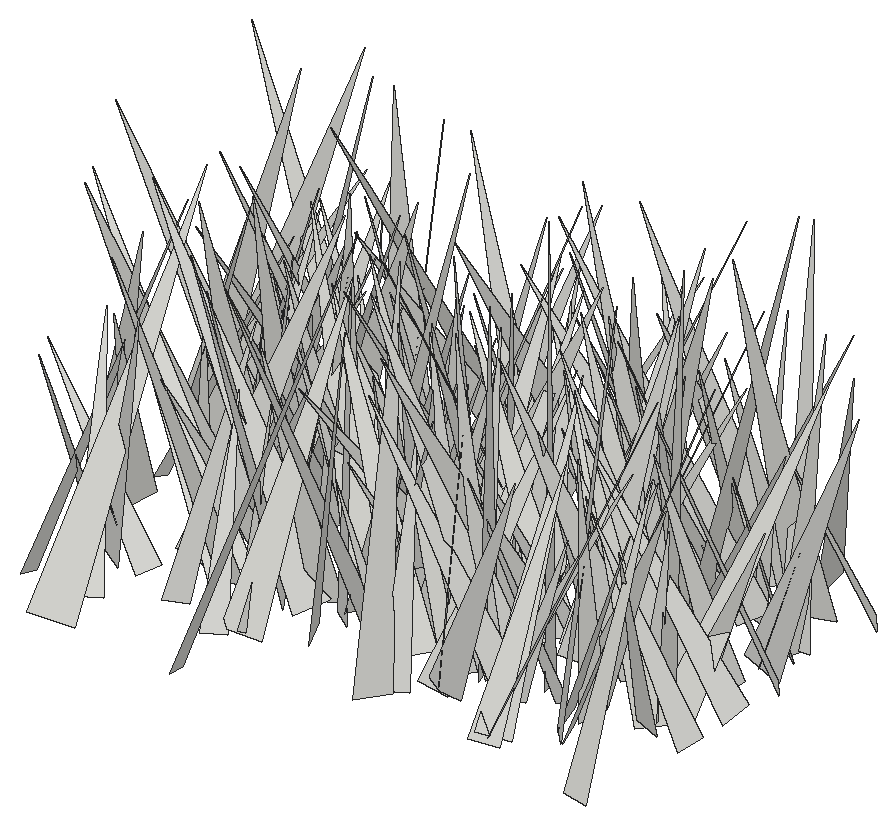
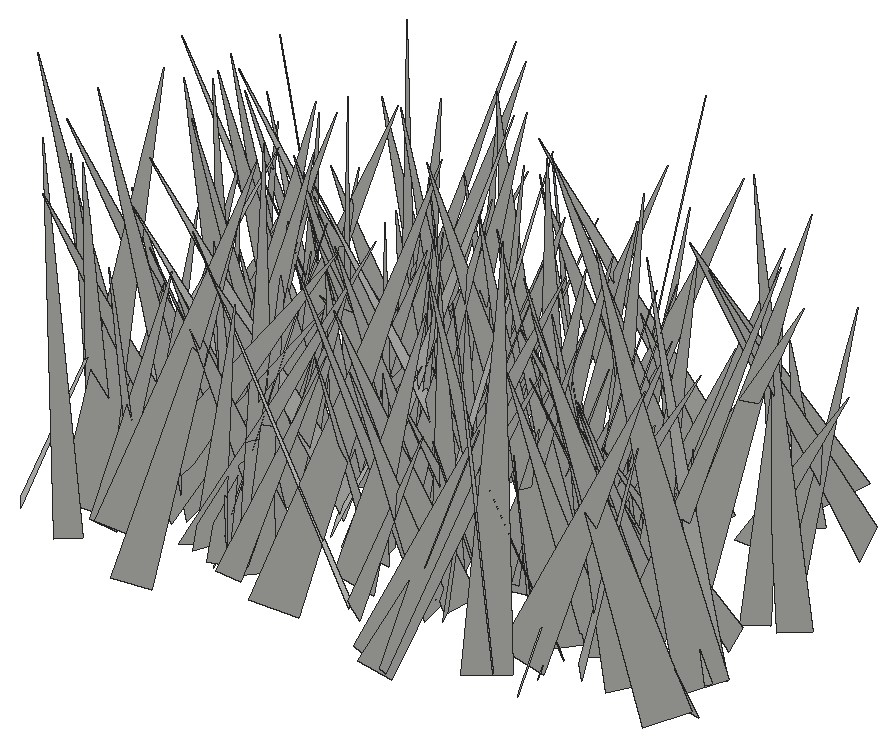
# SketchUp Ruby script. Lengths in inches.
U = 1.inch
M = Sketchup.active_model
def pt(a) = Geom::Point3d.new(a.map { |v| v * U })
def face(e, loops, mat)
  f = e.add_face(loops[0].map { |a| pt(a) })
  loops[1..].each { |l| e.add_face(l.map { |a| pt(a) }).erase! }
  f.material = f.back_material = mat if mat
  f
end
# faces: each face lists its corners as indices into pts; further lists are holes
def faces(e, pts, list, mat = nil) = list.each { |f| face(e, (f[0].is_a?(Array) ? f : [f]).map { |l| l.map { |i| pts[i] } }, mat) }
# xy, xz, yz: faces in a plane at the given z, y or x. An outline is a flat list of corners, or four numbers for a rectangle; further outlines are holes
def ring(l) = l.size == 4 ? [[l[0], l[1]], [l[2], l[1]], [l[2], l[3]], [l[0], l[3]]] : l.each_slice(2).to_a
def flat(e, list, mat, &to3) = list.each { |f| face(e, (f[0].is_a?(Array) ? f : [f]).map { |l| ring(l).map { |u, v| to3.(u, v) } }, mat) }
def xy(e, z, list, mat = nil) = flat(e, list, mat) { |x, y| [x, y, z] }
def xz(e, y, list, mat = nil) = flat(e, list, mat) { |x, z| [x, y, z] }
def yz(e, x, list, mat = nil) = flat(e, list, mat) { |y, z| [x, y, z] }
def lines(e, pts, list) = list.each { |a, b| e.add_line(pt(pts[a]), pt(pts[b])) }
# prism: a flat outline (further loops are holes) pulled along v
def prism(e, loops, v, mat = nil)
  f = face(e, loops, mat); d = Geom::Vector3d.new(v.map { |x| x * U })
  f.pushpull(f.normal.samedirection?(d) ? d.length : -d.length)
end
def box(e, o, s, mat = nil) = prism(e, [[o, [o[0] + s[0], o[1], o[2]], [o[0] + s[0], o[1] + s[1], o[2]], [o[0], o[1] + s[1], o[2]]]], [0, 0, s[2]], mat)
def at(x, y, z, deg = 0) = Geom::Transformation.translation(pt([x, y, z])) * Geom::Transformation.rotation(ORIGIN, Z_AXIS, deg.degrees)
def axes(o, x, y, z) = Geom::Transformation.new([*x, 0, *y, 0, *z, 0, *pt(o).to_a, 1])
def part(name) = M.definitions.add(name)
# library, detail: a bought-in or finely detailed component or shape, given as its bounding box
def library(name, o, s) = part(name).tap { |d| box(d.entities, o, s) }
def detail(e, o, s) = box(e.add_group.entities, o, s)
def put(e, d, t, mat = nil) = e.add_instance(d, t).tap { |i| i.material = mat if mat }
def group(e, t, mat = nil) = e.add_group.tap { |g| g.transformation = t; g.material = mat if mat }.entities
root = M.entities
c1 = part("fur_instance\#9")
p = [[0.8125,0,1.79],[0.67,-0.02,1.48],[0,-0.11,0],[0,0.11,0]]
faces(c1.entities,p,[[0,1,2,3]])
put(root,c1,axes([550.24,70.07,-21.86],[1.54833,5.59255,0.52827],[5.59137,-1.58705,0.41342],[-0.54067,-0.39706,5.78818]))
put(root,c1,axes([542.11,73.05,-21.86],[2.36521,-5.47601,0.71506],[-5.30162,-2.03369,1.96193],[1.54624,1.40343,5.6331]))
put(root,c1,axes([527.13,73.47,-21.86],[-1.49518,-5.85947,1.8909],[-5.5495,2.12534,2.19783],[2.66683,1.13753,5.63369]))
put(root,c1,axes([526.43,74.02,-21.86],[-1.58112,-4.73276,0.31075],[-4.65779,1.61119,0.83937],[0.89473,0.02406,4.91878]))
put(root,c1,axes([534.03,68.6,-21.86],[7.42778,3.7642,0.92799],[3.25227,-7.14156,2.93652],[-2.11023,2.24305,7.79217]))
put(root,c1,axes([528.46,70.68,-21.86],[-3.1637,4.01487,0.30871],[3.99884,3.17867,-0.35895],[0.47305,-0.01931,5.09895]))
put(root,c1,axes([540.15,72.93,-21.86],[-3.79704,-0.30553,0.54536],[-0.26679,3.82814,0.28712],[0.56533,-0.2455,3.79848]))
put(root,c1,axes([533.78,74.87,-21.66],[-6.24986,-4.52728,1.84324],[-4.17742,6.50052,1.80193],[2.5383,-0.44892,7.504]))
put(root,c1,axes([533.45,71.37,-21.86],[-2.96108,3.10315,0.36366],[3.04624,2.97875,-0.6142],[0.69442,0.16515,4.24503]))
put(root,c1,axes([540.63,71.06,-21.66],[-7.20595,2.28011,2.02761],[1.9171,7.42879,-1.54068],[2.37378,0.922,7.39939]))
put(root,c1,axes([528.7,68.4,-21.66],[-6.04626,5.73242,0.3376],[5.11125,5.59588,-3.47751],[2.61721,2.31459,7.57131]))
put(root,c1,axes([540.77,72.05,-21.86],[-3.00951,3.51493,1.30262],[3.55292,3.20728,-0.44587],[1.1951,-0.68362,4.60577]))
put(root,c1,axes([545.4,71.17,-21.86],[-2.46279,4.53865,0.90199],[4.34757,2.61941,-1.3098],[1.58479,-0.13272,4.99491]))
put(root,c1,axes([546.58,74.19,-21.86],[5.4983,0.81734,0.21266],[0.84397,-5.26527,-1.58403],[0.03145,-1.59793,5.32824]))
put(root,c1,axes([529.1875,73.16,-21.66],[-2.95637,3.32548,0.26078],[3.10336,2.61427,1.84435],[-1.22309,-1.40488,4.04936]))
put(root,c1,axes([536.14,73.47,-21.86],[5.56182,2.46032,2.03104],[2.73268,-5.78042,-0.48104],[-1.64644,-1.28288,6.06264]))
put(root,c1,axes([537.61,74.86,-21.66],[-2.28095,-6.51713,0.89519],[-6.46928,2.05047,-1.55597],[-1.19279,1.34151,6.72716]))
put(root,c1,axes([534.28,71.76,-21.66],[1.52611,3.71718,0.33458],[3.41655,-1.5369,1.49113],[-1.50217,0.28087,3.73135]))
put(root,c1,axes([543.6,74.67,-21.66],[-5.93019,0.58333,0.46706],[0.68124,5.75556,1.46115],[0.30714,-1.50292,5.77689]))
put(root,c1,axes([526.02,70.53,-21.66],[6.68377,2.4417,1.0502],[1.89436,-6.36953,2.75283],[-1.86446,2.28139,6.56175]))
put(root,c1,axes([531.72,74.51,-21.86],[-1.62801,-6.13851,1.48062],[-6.15059,1.19536,-1.80699],[-1.42958,1.84764,6.08822]))
put(root,c1,axes([538.4,74.24,-21.86],[5.46664,-0.56538,0.68203],[-0.51758,-5.49848,-0.40957],[-0.71898,-0.34055,5.48051]))
put(root,c1,axes([549.08,75.46,-21.86],[-0.66532,-4.77379,0.4836],[-4.67341,0.75535,1.0268],[1.0873,0.32553,4.70929]))
put(root,c1,axes([543.11,75.41,-21.66],[-6.87965,3.10007,2.46286],[3.78941,6.58637,2.29475],[1.14737,-3.16466,7.18848]))
put(root,c1,axes([545.05,72.13,-21.86],[6.48449,2.8801,0.19854],[2.8437,-6.45643,0.78158],[-0.49773,0.63448,7.05214]))
put(root,c1,axes([534.21,71.93,-21.86],[-2.25135,6.36064,1.32657],[6.19225,2.52565,-1.60099],[1.96812,-0.67041,6.55463]))
put(root,c1,axes([531.03,72.31,-21.86],[-4.17558,2.72173,1.55923],[2.19552,4.39009,-1.78362],[2.24025,0.77057,4.65424]))
put(root,c1,axes([546.375,75.9,-21.66],[0.60809,-6.43634,0.77652],[-5.71222,-0.16309,3.1214],[3.06594,0.97271,5.66154]))
put(root,c1,axes([538.57,75.5,-21.86],[-2.50316,-5.2047,1.47138],[-5.2002,2.76171,0.92225],[1.48721,0.89649,5.70124]))
put(root,c1,axes([535.08,75.55,-21.86],[1.51569,-5.39227,1.25729],[-5.41404,-1.71643,-0.83467],[-1.15995,0.96539,5.5387]))
put(root,c1,axes([542.17,78.35,-21.66],[-7.59167,-1.95799,2.55179],[-0.44126,7.11339,4.14535],[3.18601,-3.68034,6.65457]))
put(root,c1,axes([547.14,74.95,-21.86],[-4.81176,0.83188,2.6308],[1.27412,5.3609,0.63523],[2.44739,-1.15538,4.84165]))
put(root,c1,axes([544.34,74.15,-21.86],[2.6099,-2.39325,0.8726],[-2.54736,-2.4537,0.88934],[-0.00348,1.24593,3.42758]))
put(root,c1,axes([542.2,75.41,-21.86],[7.38345,1.68053,2.79244],[2.22073,-7.65548,-1.26461],[-2.38543,-1.92527,7.46594]))
put(root,c1,axes([524.36,76.62,-21.86],[0.1957,-7.90399,1.09327],[-7.43409,0.21668,2.89722],[2.89871,1.0893,7.35646]))
put(root,c1,axes([541.43,73.73,-21.86],[-4.16278,-2.64249,2.71758],[-3.23685,4.57857,-0.50613],[1.97251,1.93665,4.90462]))
put(root,c1,axes([539.58,76.72,-21.66],[-4.13984,-2.04423,0.54277],[-1.65039,3.86825,1.98107],[1.32277,-1.57147,4.17043]))
put(root,c1,axes([545.96,74.75,-21.66],[-1.77005,-3.87903,0.89181],[-3.77258,1.32393,-1.7292],[-1.26879,1.475,3.89741]))
put(root,c1,axes([542.43,75,-21.86],[1.19646,-6.35488,2.45253],[-6.76034,-1.41301,-0.36331],[-0.83491,2.33448,6.45631]))
put(root,c1,axes([534.95,75.13,-21.86],[-7.09229,4.18803,1.11711],[4.32642,6.70959,2.31334],[-0.26383,-2.55536,7.90497]))
put(root,c1,axes([551,75.46,-21.86],[-4.51725,1.3418,0.80765],[1.52463,4.33149,1.33117],[0.35811,-1.51528,4.52039]))
put(root,c1,axes([538.92,76.18,-21.86],[6.67439,0.3641,2.55328],[0.99441,-6.8993,-1.61558],[-2.3797,-1.86182,6.48614]))
put(root,c1,axes([547.3125,72.91,-21.66],[5.31201,5.41879,2.20999],[5.24419,-5.73235,1.45032],[-2.59727,-0.49162,7.44831]))
put(root,c1,axes([539.46,75.26,-21.86],[0.1838,-6.38239,2.38865],[-6.46729,0.58989,2.0738],[2.14821,2.32195,6.03888]))
put(root,c1,axes([531.91,76.76,-21.86],[-1.86711,-6.21996,0.83765],[-6.21183,1.95621,0.67975],[0.89595,0.60083,6.45848]))
put(root,c1,axes([545.6,71.44,-21.66],[-5.23053,3.77379,0.03544],[3.44734,4.80229,-2.57973],[1.53577,2.07308,5.91142]))
put(root,c1,axes([537.19,75,-21.86],[3.94564,1.0984,0.79467],[1.2,-3.96752,-0.47419],[-0.63087,-0.67703,4.06813]))
put(root,c1,axes([547.25,73.51,-21.86],[6.72288,3.05704,0.61475],[3.02645,-6.7488,0.46346],[-0.75102,0.16938,7.37074]))
put(root,c1,axes([541.33,75.17,-21.86],[-7.00283,2.97011,1.6591],[3.21934,7.01289,1.03394],[1.10002,-1.61605,7.53606]))
put(root,c1,axes([531.41,76.87,-21.86],[1.40326,-4.201,0.43994],[-3.89786,-1.46649,-1.57071],[-1.62745,-0.10993,4.1413]))
put(root,c1,axes([525.7,77.09,-21.86],[4.86782,-2.47433,0.4659],[-2.27673,-4.75873,-1.48527],[-1.07512,-1.1257,5.25471]))
put(root,c1,axes([539.97,74.31,-21.66],[-3.49983,5.63032,0.78088],[5.54982,3.18646,1.89866],[-1.22869,-1.64469,6.35172]))
put(root,c1,axes([530.04,74.71,-21.66],[-0.29437,7.39176,2.68978],[7.28817,1.26884,-2.68928],[2.95898,-2.3899,6.89148]))
put(root,c1,axes([536.23,74.91,-21.86],[3.38997,4.6985,2.258],[4.82742,-3.84601,0.75539],[-1.96736,-1.34115,5.74432]))
put(root,c1,axes([531.46,74.75,-21.66],[-4.54084,5.90887,0.08971],[5.53212,4.21055,2.68494],[-2.07809,-1.7025,6.95162]))
put(root,c1,axes([543.1,75.74,-21.66],[3.75203,3.55416,0.24846],[3.4305,-3.50645,-1.64561],[0.96201,-1.35805,4.89916]))
put(root,c1,axes([527.87,78.71,-21.86],[3.52912,-6.81057,1.30534],[-6.45742,-3.76145,-2.16695],[-2.52774,0.10047,7.35818]))
put(root,c1,axes([542.04,75.62,-21.86],[-4.89428,-1.48699,1.50253],[-1.73277,4.99254,-0.70337],[1.21087,1.13406,5.0666]))
put(root,c1,axes([549.18,75.6875,-21.86],[-2.40654,5.51072,1.54274],[5.60544,1.9331,1.83892],[-1.15197,-2.10585,5.72519]))
put(root,c1,axes([546.9375,77.85,-21.66],[2.35436,-6.19743,2.05043],[-5.78585,-2.99044,-2.39512],[-3.02263,0.89697,6.18179]))
put(root,c1,axes([536.84,80.09,-21.66],[-5.34969,-3.46152,0.37635],[-2.75195,4.62606,3.43064],[2.1332,-2.713,5.36954]))
put(root,c1,axes([539.41,77.39,-21.86],[0.94706,-3.59902,0.23008],[-3.53322,-0.8783,0.80484],[0.72266,0.42244,3.63347]))
put(root,c1,axes([542.1,74.87,-21.86],[-5.67085,1.89535,1.35099],[1.57668,5.74544,-1.44226],[1.71219,0.98676,5.80265]))
put(root,c1,axes([547.97,76.98,-21.86],[0.94774,-3.5048,1.15841],[-3.67796,-0.79512,0.60341],[0.31324,1.26803,3.58018]))
put(root,c1,axes([541.87,72.79,-21.66],[-5.06896,3.36354,0.19703],[2.56301,4.08037,-3.71862],[2.18706,3.01393,4.81452]))
put(root,c1,axes([532.12,77.16,-21.86],[6.22111,3.48137,1.76986],[3.77865,-6.20685,-1.07301],[-0.98698,-1.81924,7.04775]))
put(root,c1,axes([550.88,78.07,-21.86],[-5.67147,0.82087,0.04901],[0.80443,5.46726,1.5178],[-0.17066,-1.50898,5.5259]))
put(root,c1,axes([530.89,76.95,-21.86],[4.00395,3.96639,1.91354],[4.25291,-4.1539,-0.28869],[-1.14309,-1.56151,5.62855]))
put(root,c1,axes([548.34,78.23,-21.66],[-6.51837,1.52305,1.37348],[1.82295,6.39951,1.5551],[0.93967,-1.84981,6.5108]))
put(root,c1,axes([544.89,75.45,-21.66],[-7.31055,-2.64435,2.80127],[-3.45475,7.15889,-2.25809],[1.70424,3.16886,7.43894]))
put(root,c1,axes([545.57,78.3,-21.86],[-0.97443,-3.66118,0.75209],[-3.71136,1.03977,0.25308],[0.44234,0.6588,3.78017]))
put(root,c1,axes([534.65,78.38,-21.86],[0.82361,-5.861,1.93807],[-5.93962,-1.28507,-1.3621],[-1.68178,1.66825,5.75972]))
put(root,c1,axes([543.45,80.0625,-21.86],[5.27025,-2.47106,0.85487],[-2.00329,-5.05203,-2.25305],[-1.68041,-1.72721,5.36707]))
put(root,c1,axes([549.67,79.29,-21.86],[-4.78026,1.17069,2.19317],[1.89155,4.79719,1.56216],[1.61324,-2.15588,4.66702]))
put(root,c1,axes([547.51,78.46,-21.86],[3.76435,-5.16952,3.38659],[-5.24976,-4.76711,-1.44149],[-3.26082,1.70703,6.23028]))
put(root,c1,axes([544.7,77.33,-21.66],[3.44666,-5.98968,2.82803],[-6.61551,-2.95389,1.80641],[0.33028,3.33943,6.67028]))
put(root,c1,axes([529.6875,77.83,-21.86],[-2.04031,-2.94511,1.87891],[-3.25881,2.38849,0.20512],[1.25863,1.41005,3.57693]))
put(root,c1,axes([536.48,75.48,-21.66],[-7.17026,0.40545,3.85637],[-0.86926,7.73252,-2.42922],[3.77894,2.54801,6.75839]))
put(root,c1,axes([530.18,80.07,-21.86],[6.98441,-2.34407,2.00985],[-1.86712,-7.16517,-1.86827],[-2.45928,-1.21733,7.12645]))
put(root,c1,axes([548.81,78.53,-21.66],[2.19638,-3.75423,0.49776],[-3.62923,-1.92217,1.51658],[1.08198,1.1735,4.07656]))
put(root,c1,axes([543.73,78.63,-21.86],[-1.12844,-4.06047,0.83548],[-3.60524,0.5338,-2.27512],[-2.04639,1.29864,3.54749]))
put(root,c1,axes([535.47,77.17,-21.66],[-2.86561,6.0597,1.12131],[6.09085,2.59686,1.53195],[-0.93747,-1.65086,6.5257]))
put(root,c1,axes([533.52,80.41,-21.86],[3.03189,-3.59681,0.02756],[-3.43565,-2.90654,-1.37057],[-1.06494,-0.8632,4.50011]))
put(root,c1,axes([549.12,76.46,-21.86],[-7.37531,-1.40171,2.74866],[-2.16749,7.42249,-2.03071],[2.19589,2.61858,7.22747]))
put(root,c1,axes([536.02,79.65,-21.86],[3.85722,-2.97975,0.1804],[-2.96484,-3.85827,-0.33622],[-0.3481,-0.15623,4.86251]))
put(root,c1,axes([534.26,78.47,-21.86],[-4.50006,-1.01814,0.39176],[-1.03948,4.50642,-0.22865],[0.331,0.31016,4.60813]))
put(root,c1,axes([539.56,81.91,-21.86],[-4.65731,-6.85842,0.0184],[-6.74044,4.58127,1.51895],[1.26677,-0.83835,8.14992]))
put(root,c1,axes([528.09,80.45,-21.86],[5.91516,-3.3432,1.65321],[-2.9566,-6.09276,-1.74243],[-2.27346,-0.77492,6.56735]))
put(root,c1,axes([535.27,78.29,-21.86],[0.75971,3.71481,1.88794],[3.89435,-1.31575,1.02184],[-1.48263,-1.55251,3.65142]))
put(root,c1,axes([538.24,78.64,-21.86],[-4.24357,2.27798,1.78244],[2.54082,4.44811,0.36434],[1.38223,-1.18292,4.80254]))
put(root,c1,axes([532.11,79.93,-21.86],[6.97183,-3.45055,1.53762],[-3.37643,-7.13932,-0.71191],[-1.69419,0.0288,7.74635]))
put(root,c1,axes([540.2,77.57,-21.86],[-6.10428,-1.79449,1.71008],[-2.20054,6.01533,-1.54278],[1.14113,2.0006,6.1727]))
put(root,c1,axes([531.71,80.39,-21.86],[-1.20375,-5.21342,0.24756],[-5.17288,1.15789,-0.76855],[-0.69453,0.4118,5.2951]))
put(root,c1,axes([543.9375,79.125,-21.86],[0.78956,-4.05986,1.16414],[-3.93825,-0.27989,1.69498],[1.52574,1.37851,3.77266]))
put(root,c1,axes([542.85,78.51,-21.86],[-4.45803,3.98436,0.74293],[4.03358,4.25341,1.39275],[-0.39655,-1.52789,5.81458]))
put(root,c1,axes([530.01,77.12,-21.86],[5.78446,0.51407,0.77192],[0.25637,-5.57234,1.78981],[-0.89129,1.73346,5.52457]))
put(root,c1,axes([535.3,83.68,-21.66],[-5.2335,-6.40482,0.23356],[-5.52847,4.66397,4.0186],[3.24225,-2.38569,7.22925]))
put(root,c1,axes([539.14,79.87,-21.86],[-2.90211,-6.23156,1.67253],[-6.44447,2.71044,-1.08359],[-0.31368,1.96803,6.78825]))
put(root,c1,axes([526.38,79.61,-21.86],[-0.14412,-3.47359,1.04669],[-3.58722,0.2928,0.47779],[0.54152,1.01518,3.44359]))
put(root,c1,axes([524.22,81.09,-21.86],[7.41722,0.99885,0.34739],[1.05742,-6.96886,-2.53978],[0.01548,-2.56338,7.04006]))
put(root,c1,axes([549.03,77.23,-21.86],[0.07577,6.70614,0.84141],[6.48392,0.16538,-1.90197],[1.90764,-0.82847,6.43122]))
put(root,c1,axes([545.5,79.54,-21.86],[-3.79672,1.89832,0.59417],[1.98792,3.66583,0.99077],[0.06937,-1.15319,4.1276]))
put(root,c1,axes([539.99,77.1,-21.86],[0.187,6.43803,0.46404],[6.40843,-0.12967,-0.78342],[0.77175,-0.48321,6.39292]))
put(root,c1,axes([527.74,79.08,-21.86],[4.06898,-3.86093,0.67624],[-3.71406,-3.48612,2.44405],[1.25293,2.20473,5.04877]))
put(root,c1,axes([550.85,80.45,-21.86],[-5.4011,-4.4458,0.12135],[-4.40164,5.31613,-1.14717],[-0.63674,0.96192,6.9008]))
put(root,c1,axes([535.85,78.33,-21.86],[3.84083,1.33111,0.88578],[1.09907,-3.87194,1.0529],[-1.16125,0.73803,3.92622]))
put(root,c1,axes([527.86,81.54,-21.86],[-7.8024,0.71377,1.7229],[1.19599,7.6017,2.26696],[1.43089,-2.46171,7.49986]))
put(root,c1,axes([544.04,79.35,-21.86],[-4.7779,-0.84592,1.0787],[-0.97294,4.84801,-0.50762],[0.9657,0.69908,4.82558]))
put(root,c1,axes([537.45,77.01,-21.86],[6.47525,4.61232,0.40047],[4.47579,-6.41261,1.48613],[-1.18373,0.98374,7.80985]))
put(root,c1,axes([542.75,77.96,-21.66],[-5.36407,2.31527,0.60969],[2.0889,5.25672,-1.5839],[1.1699,1.22955,5.6236]))
put(root,c1,axes([544.68,80.56,-21.86],[1.6475,-3.20979,0.84583],[-3.31321,-1.64761,0.20101],[-0.20196,0.8456,3.6023]))
put(root,c1,axes([549.58,81.11,-21.86],[1.03631,-6.95808,1.71035],[-6.57848,-0.23906,3.0134],[2.83968,1.98547,6.35675]))
put(root,c1,axes([537.22,80.57,-21.66],[1.67696,-6.87357,2.26471],[-6.67493,-0.57073,3.21041],[2.79647,2.7596,6.30488]))
put(root,c1,axes([538.59,81.03,-21.86],[5.52429,1.58059,2.16664],[1.98524,-5.74559,-0.8703],[-1.80317,-1.48335,5.67966]))
put(root,c1,axes([529.71,81.19,-21.86],[7.30646,0.41261,0.41525],[0.46932,-7.23653,-1.06747],[-0.34987,-1.09065,7.23983]))
put(root,c1,axes([536.02,80.98,-21.86],[-0.35504,-4.51922,1.36303],[-4.31721,-0.2418,-1.92625],[-1.90863,1.3876,4.10353]))
put(root,c1,axes([538.7,78.41,-21.86],[-1.23708,6.4323,0.84499],[6.38548,1.35924,-0.99849],[1.14637,-0.62994,6.47363]))
put(root,c1,axes([545.5,81.91,-21.66],[4.05773,-0.76512,0.97615],[-0.40955,-3.97873,-1.41614],[-1.1707,-1.26007,3.87881]))
put(root,c1,axes([525.39,78.56,-21.66],[4.79921,1.03907,0.41248],[0.79797,-4.45725,1.94381],[-0.78297,1.82633,4.50929]))
put(root,c1,axes([533.67,80.87,-21.86],[5.98361,0.11352,0.76596],[0.13466,-6.02993,-0.15823],[-0.76252,-0.17402,5.9826]))
put(root,c1,axes([537.23,80.42,-21.66],[-6.20853,-2.44848,0.56631],[-2.51301,6.03462,-1.45936],[-0.02325,1.56521,6.51238]))
put(root,c1,axes([528.33,78.9375,-21.86],[0.97806,5.36378,0.25201],[5.36787,-0.98334,0.09641],[-0.14015,-0.23057,5.45137]))
put(root,c1,axes([535.39,81.74,-21.86],[4.53528,-3.04969,1.17101],[-3.07507,-4.66168,-0.23091],[-1.10265,0.45689,5.46041]))
put(root,c1,axes([541.24,80.64,-21.86],[-4.27231,-1.94809,0.06255],[-1.87913,4.07681,-1.37844],[-0.51754,1.27912,4.48861]))
put(root,c1,axes([530.96,83.12,-21.66],[-0.84326,-5.89202,0.02664],[-5.53518,0.78295,-2.04363],[-2.01949,0.3143,5.59022]))
put(root,c1,axes([549.2,81.73,-21.86],[4.10425,1.09153,0.3293],[1.14011,-3.92312,-1.20584],[0.00571,-1.24998,4.07214]))
put(root,c1,axes([543.22,80.04,-21.86],[1.96643,7.28816,1.86053],[7.47956,-1.69089,-1.28167],[0.79683,-2.11408,7.43918]))
put(root,c1,axes([535.78,79.3,-21.86],[3.9731,1.20771,1.01378],[0.70264,-3.81635,1.79266],[-1.41159,1.49959,3.74573]))
put(root,c1,axes([529.6875,82.71,-21.66],[2.97269,-7.01093,0.81561],[-6.80259,-2.60982,2.35986],[1.88234,1.64042,7.24024]))
put(root,c1,axes([543.67,80.74,-21.86],[-3.45745,4.3845,0.64107],[4.38114,3.2607,1.32749],[-0.66366,-1.31634,5.42361]))
put(root,c1,axes([544.2,83.3,-21.86],[-0.85203,-5.57664,0.61964],[-5.3803,0.98986,1.51043],[1.59225,0.36067,5.43539]))
put(root,c1,axes([542.95,82.36,-21.86],[6.79044,-4.4332,0.71146],[-4.48312,-6.76549,0.63187],[-0.24718,0.91888,8.0848]))
put(root,c1,axes([527.43,79.67,-21.66],[5.0446,1.96996,1.21492],[1.59207,-5.06819,1.60732],[-1.6799,1.1124,5.17158]))
put(root,c1,axes([534.01,80.46,-21.86],[-2.66965,3.73747,0.14274],[3.69986,2.61324,0.77338],[-0.54785,-0.56423,4.52743]))
put(root,c1,axes([533.875,81.375,-21.86],[-5.56985,2.38046,0.65327],[2.45077,5.52546,0.76123],[0.29505,-0.95874,6.00918]))
put(root,c1,axes([544.21,79,-21.86],[5.76242,3.50846,0.12226],[3.39302,-5.62636,1.53663],[-0.90093,1.2508,6.56914]))
put(root,c1,axes([545.87,80.82,-21.66],[-0.49595,7.7495,2.67586],[7.77568,-0.40515,2.61451],[-2.59882,-2.6911,7.31198]))
put(root,c1,axes([544.01,78.06,-21.66],[-5.33853,3.8285,0.2094],[3.37353,4.86067,-2.86257],[1.82225,2.21756,5.91295]))
put(root,c1,axes([549.875,82.33,-21.86],[-2.17535,-3.01047,0.60266],[-3.06621,2.16789,-0.23847],[0.15643,0.62897,3.70651]))
put(root,c1,axes([524.37,81.61,-21.86],[6.94828,-4.27135,1.74082],[-4.55894,-6.83788,1.41876],[-0.70067,2.13364,8.03182]))
put(root,c1,axes([526.25,83.69,-21.66],[0.97454,-6.53217,0.4424],[-5.83998,-0.6651,3.04417],[2.95966,0.83851,5.86106]))
put(root,c1,axes([529.08,84.63,-21.66],[-5.93761,-4.29126,0.84113],[-3.95201,5.87307,2.0655],[1.8719,-1.21235,7.02879]))
put(root,c1,axes([544.39,83.7,-21.86],[-3.97091,-3.72473,0.66515],[-3.58252,4.01146,1.07602],[1.21718,-0.34456,5.33703]))
put(root,c1,axes([541.55,79.375,-21.66],[7.40987,3.38689,0.1989],[3.26816,-7.25381,1.76579],[-0.91088,1.52574,7.95356]))
put(root,c1,axes([529.02,80.14,-21.86],[7.21368,2.51232,2.17903],[2.05011,-7.45745,1.81123],[-2.61859,1.08246,7.42081]))
put(root,c1,axes([538.5,81.67,-21.86],[-0.50007,3.75556,1.02909],[3.87876,0.38868,0.46638],[-0.34425,-1.07612,3.75989]))
put(root,c1,axes([539.24,86.44,-21.86],[4.97759,-6.71856,0.2944],[-6.18791,-4.7191,-3.07278],[-2.63353,-1.61035,7.77647]))
put(root,c1,axes([542.67,82.05,-21.66],[3.6305,3.98779,0.322],[3.84064,-3.3521,-1.78874],[1.12055,-1.43096,5.08758]))
put(root,c1,axes([534.94,80.61,-21.86],[1.96135,3.70682,0.36248],[3.45553,-1.96392,1.38604],[-1.38968,0.34826,3.95807]))
put(root,c1,axes([542.39,84.5,-21.66],[6.00758,0.21792,0.49644],[0.387,-5.59183,-2.22857],[-0.3797,-2.2514,5.58318]))
put(root,c1,axes([528.79,86.17,-21.66],[-5.78164,-4.6449,0.78576],[-4.06196,5.54542,2.89287],[2.386,-1.8147,6.82889]))
put(root,c1,axes([541.22,84.92,-21.86],[7.15666,-2.1147,0.99823],[-1.83229,-7.06792,-1.83669],[-1.45298,-1.50292,7.233]))
put(root,c1,axes([549.73,82.44,-21.86],[5.90361,-0.69248,2.28384],[-0.937,-6.27702,0.51884],[-2.19488,0.81708,5.9214]))
put(root,c1,axes([542.72,85.21,-21.86],[-1.15105,-5.30671,0.17],[-5.09537,1.15297,1.49093],[1.49242,-0.15644,5.22142]))
put(root,c1,axes([541.35,84.82,-21.66],[5.83634,-0.86723,1.56304],[-0.35494,-5.79341,-1.88904],[-1.75191,-1.71533,5.58985]))
put(root,c1,axes([528.32,83.36,-21.86],[-3.38614,-3.10021,1.02366],[-3.22386,3.40798,-0.34286],[0.51569,0.94841,4.57818]))
put(root,c1,axes([534.35,83.2,-21.86],[-3.28529,-1.60429,1.12724],[-1.66632,3.44368,0.04462],[1.03333,0.45264,3.6558]))
put(root,c1,axes([543.97,84.9,-21.66],[-6.77007,0.71674,0.61078],[0.8862,6.3486,2.37288],[0.31848,-2.42944,6.38099]))
put(root,c1,axes([548.71,85.02,-21.86],[1.61042,-7.88282,1.5376],[-7.97737,-1.75156,-0.62458],[-0.92985,1.37466,8.02136]))
put(root,c1,axes([534.4,82.29,-21.86],[5.41003,-2.25588,0.78895],[-2.38957,-5.13634,1.69936],[-0.03699,1.87321,5.60977]))
put(root,c1,axes([528.38,82.05,-21.86],[-0.72846,5.64896,1.65026],[5.62241,1.15927,-1.48642],[1.73859,-1.38206,5.49837]))
put(root,c1,axes([545.82,85.23,-21.86],[-0.77388,-5.77446,0.46112],[-5.72229,0.83441,0.84559],[0.90132,0.33953,5.76439]))
put(root,c1,axes([546.32,83.61,-21.66],[-2.71557,-5.16024,0.69315],[-4.67023,2.06855,-2.89705],[-2.30163,1.89099,5.06058]))
put(root,c1,axes([546.38,81.64,-21.66],[6.37696,0.70596,0.43543],[0.57496,-6.19552,1.62437],[-0.59783,1.57187,6.20688]))
put(root,c1,axes([545.54,82.59,-21.86],[8.05424,1.38868,1.7961],[1.29513,-8.24767,0.56905],[-1.86468,0.26973,8.15325]))
put(root,c1,axes([539.23,81.06,-21.86],[1.91748,5.33638,0.31642],[5.10909,-1.9283,1.55969],[-1.57297,0.24194,5.4517]))
put(root,c1,axes([542.94,84.98,-21.86],[-5.52316,-3.7636,0.965],[-3.71814,5.60658,0.58551],[1.12752,0.05244,6.65787]))
put(root,c1,axes([547.43,83.44,-21.66],[-2.51256,7.06983,2.10699],[6.38069,0.96553,4.36915],[-3.70253,-3.13371,6.09968]))
put(root,c1,axes([523.4,83.28,-21.86],[4.19059,5.13354,0.34706],[4.85008,-3.79176,-2.47669],[1.71767,-1.81771,6.14657]))
put(root,c1,axes([531.56,82.01,-21.66],[2.74983,3.97442,1.3241],[3.39736,-3.04242,2.07665],[-2.45097,0.24187,4.36407]))
put(root,c1,axes([529.61,82.8,-21.86],[2.54826,3.20038,0.28055],[3.20908,-2.5526,-0.02947],[-0.15164,-0.23787,4.09087]))
put(root,c1,axes([541.13,83.35,-21.66],[5.01849,-2.22986,0.6447],[-2.32023,-4.77497,1.54574],[0.06662,1.67347,5.26955]))
put(root,c1,axes([535.53,82.82,-21.66],[2.61038,6.20008,1.07332],[6.21386,-2.35716,-1.49626],[0.99041,-1.55238,6.55868]))
put(root,c1,axes([541.64,85.94,-21.66],[1.73038,-3.85975,0.19684],[-3.59553,-1.68683,-1.46882],[-1.41726,-0.43309,3.96667]))
put(root,c1,axes([530.71,85.48,-21.86],[5.1556,-5.75467,2.21602],[-5.90961,-5.43588,-0.36737],[-1.76168,1.39363,7.71761]))
put(root,c1,axes([546.59,85.75,-21.66],[2.25381,-7.00366,2.80187],[-6.80723,-3.14832,-2.39397],[-3.25014,1.7373,6.957]))
put(root,c1,axes([537.4,84.62,-21.86],[5.77692,4.11347,0.10405],[3.90568,-5.42514,-2.37018],[1.29504,-1.98782,6.68399]))
put(root,c1,axes([550.63,86.05,-21.86],[-3.47143,-2.84551,0.09651],[-2.81271,3.45107,0.57956],[0.4415,-0.38766,4.45106]))
put(root,c1,axes([534.25,87.45,-21.66],[-1.51333,-7.7582,0.0595],[-7.60064,1.47034,-1.59746],[-1.5568,0.36304,7.74132]))
put(root,c1,axes([547.79,87,-21.86],[6.93671,-0.62868,0.23505],[-0.51232,-6.5363,-2.3628],[-0.4336,-2.33453,6.55213]))
put(root,c1,axes([549.61,82.85,-21.86],[1.24745,7.40868,1.63783],[7.39275,-1.56046,1.42803],[-1.70827,-1.34297,7.376]))
put(root,c1,axes([547.4,85.56,-21.86],[0.47741,-4.86513,1.33169],[-4.92648,-0.73691,-0.92606],[-1.08291,1.20759,4.79999]))
put(root,c1,axes([537.9375,83.71,-21.66],[-2.07893,6.71015,1.41675],[6.64432,1.60395,2.15305],[-1.69892,-1.93817,6.68674]))
put(root,c1,axes([537.01,84.86,-21.86],[0.7235,3.49331,2.20248],[3.65755,-1.58024,1.30491],[-1.91742,-1.69623,3.32022]))
put(root,c1,axes([534.85,83.07,-21.86],[5.29795,0.17393,1.896],[-0.4687,-5.31448,1.7972],[-1.84537,1.84915,4.98684]))
put(root,c1,axes([533.875,87.63,-21.86],[2.44843,-5.51273,0.60157],[-4.8536,-2.44839,-2.68234],[-2.6823,-0.60174,5.40279]))
put(root,c1,axes([523.96,84.08,-21.86],[6.06814,-4.77445,2.10475],[-5.2154,-5.64781,2.22478],[-0.15808,3.05854,7.39379]))
put(root,c1,axes([531.01,84.6875,-21.86],[5.52113,3.74347,2.2115],[4.00437,-5.77059,-0.2291],[-1.6939,-1.44011,6.66663]))
put(root,c1,axes([547.47,83.59,-21.86],[2.35955,4.93164,1.36493],[4.86886,-2.62618,1.07189],[-1.57426,-0.73054,5.36093]))
put(root,c1,axes([544.13,88.13,-21.86],[4.15216,-5.25606,0.30062],[-4.95254,-4.0295,-2.04756],[-1.78575,-1.04593,6.37763]))
put(root,c1,axes([530.36,84.02,-21.86],[-2.68904,7.46116,1.26428],[7.06219,1.99214,3.26422],[-2.71897,-2.20471,7.22805]))
put(root,c1,axes([543.69,84.44,-21.86],[-4.9618,2.41645,1.1014],[2.44275,5.06865,-0.11597],[1.04177,-0.37582,5.51772]))
